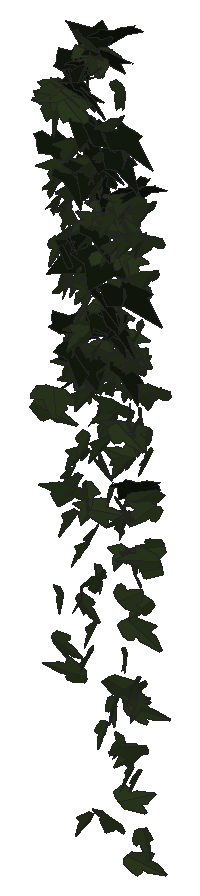
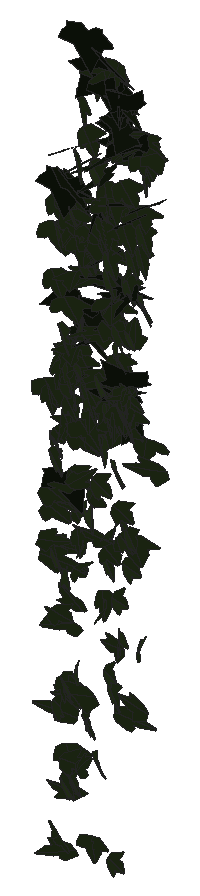
# SketchUp Ruby script. Lengths in millimetres.
U = 1.mm
M = Sketchup.active_model
def pt(a) = Geom::Point3d.new(a.map { |v| v * U })
def face(e, loops, mat)
  f = e.add_face(loops[0].map { |a| pt(a) })
  loops[1..].each { |l| e.add_face(l.map { |a| pt(a) }).erase! }
  f.material = f.back_material = mat if mat
  f
end
# faces: each face lists its corners as indices into pts; further lists are holes
def faces(e, pts, list, mat = nil) = list.each { |f| face(e, (f[0].is_a?(Array) ? f : [f]).map { |l| l.map { |i| pts[i] } }, mat) }
# xy, xz, yz: faces in a plane at the given z, y or x. An outline is a flat list of corners, or four numbers for a rectangle; further outlines are holes
def ring(l) = l.size == 4 ? [[l[0], l[1]], [l[2], l[1]], [l[2], l[3]], [l[0], l[3]]] : l.each_slice(2).to_a
def flat(e, list, mat, &to3) = list.each { |f| face(e, (f[0].is_a?(Array) ? f : [f]).map { |l| ring(l).map { |u, v| to3.(u, v) } }, mat) }
def xy(e, z, list, mat = nil) = flat(e, list, mat) { |x, y| [x, y, z] }
def xz(e, y, list, mat = nil) = flat(e, list, mat) { |x, z| [x, y, z] }
def yz(e, x, list, mat = nil) = flat(e, list, mat) { |y, z| [x, y, z] }
def lines(e, pts, list) = list.each { |a, b| e.add_line(pt(pts[a]), pt(pts[b])) }
# prism: a flat outline (further loops are holes) pulled along v
def prism(e, loops, v, mat = nil)
  f = face(e, loops, mat); d = Geom::Vector3d.new(v.map { |x| x * U })
  f.pushpull(f.normal.samedirection?(d) ? d.length : -d.length)
end
def box(e, o, s, mat = nil) = prism(e, [[o, [o[0] + s[0], o[1], o[2]], [o[0] + s[0], o[1] + s[1], o[2]], [o[0], o[1] + s[1], o[2]]]], [0, 0, s[2]], mat)
def at(x, y, z, deg = 0) = Geom::Transformation.translation(pt([x, y, z])) * Geom::Transformation.rotation(ORIGIN, Z_AXIS, deg.degrees)
def axes(o, x, y, z) = Geom::Transformation.new([*x, 0, *y, 0, *z, 0, *pt(o).to_a, 1])
def part(name) = M.definitions.add(name)
# library, detail: a bought-in or finely detailed component or shape, given as its bounding box
def library(name, o, s) = part(name).tap { |d| box(d.entities, o, s) }
def detail(e, o, s) = box(e.add_group.entities, o, s)
def put(e, d, t, mat = nil) = e.add_instance(d, t).tap { |i| i.material = mat if mat }
def group(e, t, mat = nil) = e.add_group.tap { |g| g.transformation = t; g.material = mat if mat }.entities
root = M.entities
M.materials.add("efeu1").color = [18, 25, 13]
M.materials.add("efeu2").color = [43, 57, 29]
c1 = part("ivyleaf_10")
p = [[0,12.8,-0.8],[-1.5,51.3,-10.9],[-4.9,51,-11.6],[-13.6,26.5,-7.3],[-13.2,15.9,-4.6],[-21.1,19.3,-7.2],
  [-29.5,16.3,-8.3],[-29.2,8.3,-6.2],[-19.7,-9.8,0.5],[-7.6,-13,4],[1,-12.2,5.8],[-0.4,51.1,-11.1],
  [-1.5,51.1,-10.9],[1,-12.4,5.9],[16.9,-12.4,3.5],[35.1,9.1,-5.1],[35,12.9,-6.1],[20.5,16.4,-4.9],
  [15.8,15,-3.8],[15.3,27.6,-7.1],[12.8,31.3,-7.8]]
faces(c1.entities,p,[[0,1,2,3,4,5,6,7,8,9,10],[11,12,0,13,14,15,16,17,18,19,20]],"efeu2")
c2 = part("ivyleaf_9")
p = [[39.1,54.8,31.7],[34.5,51.8,30.2],[-5.3,25.2,17.3],[-17.9,28.3,20.9],[-21.6,21.7,17],[-20.2,4.3,5.3],
  [-22.9,-0.3,2.5],[-17.1,-4,-0.6],[-2,-2.1,-1.2],[-0.7,-15.4,-10.1],[16.6,-22.3,-16.7],[21.1,-15.1,-12.5],
  [32.7,-10.7,-11],[46.1,-1.8,-6.6],[30.8,11.2,3.8]]
faces(c2.entities,p,[[0,1,2,3,4,5,6,7,8,9,10,11,12,13,14]],"efeu1")
put(root,c1,axes([1236.6,996.8,859],[-0.48434,-0.01854,-0.67596],[1.27265,-0.11431,-0.24861],[-0.1914,-0.71317,0.05742]))
put(root,c1,axes([1267.7,996.5,1433.3],[-0.73071,-0.64843,0.24389],[-0.04626,-0.26606,-0.74563],[1.31768,-0.36892,0.10907]))
put(root,c1,axes([1262.1,1002.8,1162.8],[0.77658,-0.63464,0.15423],[0.15396,-0.13134,-0.75449],[1.23344,0.41597,-0.00293]))
put(root,c2,axes([1251,1002.6,1352.9],[0.2551,-0.72169,-0.24865],[0.08886,0.25974,-0.72869],[1.45004,0.11105,0.0884]))
put(root,c1,axes([1269.6,998,1254.6],[0.07758,-0.76332,-0.07843],[0.03185,0.0794,-0.76412],[1.46005,0.03882,0.02083]))
put(root,c1,axes([1278.6,1010,717.3],[-1.12301,-0.45413,0.18457],[-0.24328,-0.1363,-0.74402],[0.90069,-0.60305,0.02917]))
put(root,c1,axes([1272.7,990.3,1291.2],[-0.0053,-0.76905,0.00236],[-0.00122,-0.00236,-0.76906],[1.46367,-0.00279,-0.00063]))
put(root,c1,axes([1247.8,1026.8,420],[-0.05358,0.0607,-0.71661],[0.97993,-0.499,-0.06249],[-0.95561,-0.5151,-0.0239]))
put(root,c1,axes([1270.7,1026.9,740.1],[0.12388,-0.62126,0.15416],[0.10876,-0.1487,-0.62337],[1.21338,0.07676,0.04014]))
put(root,c1,axes([1270.5,987.4,1404.9],[0.66757,-0.69995,-0.15253],[0.11635,0.19846,-0.77014],[1.35844,0.32697,0.14092]))
put(root,c1,axes([1285.4,992.2,1461.8],[1.00596,0.26839,-0.54166],[-0.95,-0.21209,-0.59217],[-0.64897,0.7265,0.02723]))
put(root,c1,axes([1297.6,1010.7,384.3],[-0.04672,-0.00322,0.68376],[-1.24545,-0.19826,-0.02443],[0.3773,-0.65485,0.00403]))
put(root,c1,axes([1255.8,994,1442.4],[-0.97704,-0.15716,-0.58973],[1.10384,0.11426,-0.53534],[0.36159,-0.77348,0.04075]))
put(root,c1,axes([1265.2,986.9,897.9],[1.3992,0.19283,0.10718],[0.18718,0.04733,-0.75977],[-0.37585,0.74144,0.02063]))
put(root,c1,axes([1264.9,1007.9,514.3],[-0.18596,-0.0466,0.72839],[0.74159,-0.62473,0.0123],[1.17458,0.38705,0.10756]))
put(root,c1,axes([1277,1007.8,1090.6],[-0.35052,-0.6667,-0.28883],[-0.17614,-0.27401,0.69151],[-1.37156,0.20558,-0.01499]))
put(root,c1,axes([1282.5,1020.9,948.5],[0.50606,-0.62103,-0.12277],[-0.07777,0.11604,-0.67551],[1.20231,0.2689,0.00798]))
put(root,c1,axes([1285.2,988.6,1322.2],[-0.86934,-0.61046,0.15935],[-0.01235,-0.19217,-0.75481],[1.2007,-0.44397,0.10761]))
put(root,c1,axes([1282.6,1027.7,729],[0.00113,-0.57979,0.27924],[0.05888,-0.27889,-0.57913],[1.22335,0.01396,0.02762]))
put(root,c1,axes([1281.4,1000.5,949.3],[0.20567,-0.46714,-0.52578],[0.14616,0.53661,-0.46098],[1.33057,0.01326,0.13191]))
put(root,c1,axes([1285.9,1001.7,1249.9],[-0.02219,-0.75998,-0.05861],[0.01802,0.05847,-0.76002],[1.45058,-0.01235,0.00854]))
put(root,c1,axes([1285.1,992.2,1459.4],[1.24855,0.43136,-0.17251],[-0.39567,0.00564,-0.7765],[-0.79071,0.67831,0.11616]))
put(root,c1,axes([1288.1,1008.4,1199.9],[-0.03972,-0.74212,-0.0126],[-0.00115,0.01262,-0.74241],[1.41261,-0.02086,-0.00096]))
put(root,c1,axes([1285.7,1012.2,668.7],[0.12431,-0.5106,0.52642],[0.19752,-0.51675,-0.5141],[1.3817,0.11981,0.02613]))
put(root,c1,axes([1291.2,1029.3,781.1],[-0.17924,-0.53573,0.39099],[-0.05732,-0.39105,-0.54307],[1.26097,-0.09393,0.03089]))
put(root,c1,axes([1280.5,1014.4,1107.4],[0.30435,-0.46144,0.60436],[0.46387,-0.55388,-0.4874],[1.37079,0.28989,0.03075]))
put(root,c1,axes([1291.8,1013.3,955.6],[-1.04393,-0.48159,-0.06748],[0.10188,0.04131,-0.72992],[0.9199,-0.5511,0.00426]))
put(root,c1,axes([1291.3,1005.5,975.5],[0.34361,-0.4942,-0.48629],[-0.00492,0.50203,-0.51115],[1.31955,0.13056,0.12472]))
put(root,c1,axes([1289.1,994.5,1234.4],[0.18803,-0.5842,-0.47304],[0.28392,0.48285,-0.56517],[1.40218,-0.01943,0.17787]))
put(root,c1,axes([1315,1007.3,986.2],[-0.75242,-0.02108,0.59441],[-1.09376,-0.1704,-0.38827],[0.29172,-0.69324,0.07736]))
put(root,c2,axes([1289.2,998.2,1185.1],[1.01041,-0.23892,-0.52743],[-0.86423,0.27219,-0.58038],[0.68375,0.69711,0.04585]))
put(root,c1,axes([1287.1,1007.1,992.1],[0.15937,-0.06374,0.73173],[0.0287,0.73646,0.06242],[-1.3976,0.00786,0.08472]))
put(root,c2,axes([1298,983.1,925.4],[0.26957,0.57002,0.50842],[0.24425,0.49198,-0.58734],[-1.43303,0.19108,-0.00447]))
put(root,c1,axes([1297.4,1009.4,737.9],[0.35226,-0.59652,-0.18005],[-0.02889,0.18345,-0.6234],[1.18554,0.18172,0.03831]))
put(root,c1,axes([1296.6,1019.9,965.4],[0.406,-0.6716,0.06352],[0.02866,-0.06187,-0.70465],[1.28357,0.21381,-0.00436]))
put(root,c1,axes([1300.5,999,1285.3],[-0.2733,-0.7494,0.01594],[-0.01021,-0.0152,-0.76303],[1.42655,-0.14368,-0.00241]))
put(root,c1,axes([1300,1019.5,1109.2],[0.02503,-0.67465,0.2926],[0.03464,-0.29226,-0.67469],[1.39914,0.01931,0.01147]))
put(root,c1,axes([1308.9,1011.7,980.1],[-0.46867,0.52454,-0.45681],[-0.36459,0.4147,0.57947],[1.27261,0.31198,-0.00222]))
put(root,c2,axes([1287.3,1009.8,1009.3],[-0.69557,-0.07879,0.68714],[1.27312,0.15724,0.37382],[-0.33453,0.76224,-0.00609]))
put(root,c2,axes([1301.2,990.1,1476.8],[0.62333,0.64045,0.36642],[0.0415,0.39232,-0.70521],[-1.40368,0.296,0.14186]))
put(root,c1,axes([1305.4,997.2,1365.4],[-0.52946,-0.69054,0.23758],[-0.07237,-0.24019,-0.74266],[1.38796,-0.27594,0.0519]))
put(root,c1,axes([1298.2,1026.1,608.2],[0.13264,-0.43926,0.49745],[0.19787,-0.48679,-0.44441],[1.24744,0.12392,0.0176]))
put(root,c1,axes([1300.2,1006.7,989.5],[0.0641,-0.16022,0.69276],[-0.27177,0.67788,0.16372],[-1.3257,-0.14672,-0.00007]))
put(root,c2,axes([1321,997.8,1195.3],[-0.81049,0.61854,0.11361],[-0.09102,0.10495,-0.7507],[-1.19344,-0.42807,-0.0199]))
put(root,c1,axes([1301.8,1016,928],[-1.11684,-0.40969,-0.16454],[0.27417,0.08102,-0.71552],[0.79426,-0.60405,0.01563]))
put(root,c1,axes([1306.2,1005.1,528.2],[0.0608,-0.47522,-0.52635],[-0.0232,0.52644,-0.47603],[1.34943,0.03046,0.01553]))
put(root,c2,axes([1292.6,1002.4,1307.7],[-0.06609,-0.77013,0.0127],[-0.0186,-0.01227,-0.77086],[1.4658,-0.03488,-0.00921]))
put(root,c1,axes([1307.3,1016,940.5],[-0.04105,-0.61766,-0.40572],[0.05295,0.40493,-0.61793],[1.40547,-0.03329,0.01143]))
put(root,c1,axes([1305.6,1027.5,116.3],[0.02412,-0.5141,0.4136],[0.1196,-0.41086,-0.51261],[1.25006,0.04923,0.04106]))
put(root,c2,axes([1295.7,989.2,1471],[1.47071,0.15477,-0.17109],[-0.32731,-0.01221,-0.78782],[-0.29267,0.79138,0.02131]))
put(root,c2,axes([1282.1,993,1451.1],[1.02002,-0.52969,0.2753],[0.43293,-0.16085,-0.75232],[1.05041,0.58066,0.04274]))
put(root,c2,axes([1296.9,996.5,1168.3],[0.55199,-0.61027,-0.36689],[-0.19549,0.35616,-0.67361],[1.34103,0.30312,0.05282]))
put(root,c2,axes([1303.6,987.9,1510.1],[-0.44831,-0.17537,0.75681],[1.161,0.44791,0.29366],[-0.91546,0.65392,0.00181]))
put(root,c2,axes([1307.4,1008.5,980.3],[-0.46016,-0.73558,0.02858],[-0.01743,-0.02707,-0.7743],[1.4009,-0.24196,-0.00025]))
put(root,c1,axes([1316.2,1025.1,692.7],[-0.46916,-0.50319,0.3595],[0.05123,-0.39538,-0.53494],[1.17586,-0.18355,0.16675]))
put(root,c2,axes([1326.4,998.3,1163.9],[-1.02599,-0.43006,0.3961],[-0.5662,-0.26206,-0.68941],[0.95795,-0.6155,0.01676]))
put(root,c1,axes([1316.3,1017.5,1152.3],[-1.0997,-0.47349,0.0296],[0.17302,-0.15629,-0.72543],[0.88618,-0.55707,0.17837]))
put(root,c1,axes([1303.7,982.4,1439.8],[0.48291,0.68445,0.326],[0.26394,0.29607,-0.72955],[-1.41851,0.2881,-0.02476]))
put(root,c1,axes([1320.2,998.4,1036.4],[-0.44478,-0.68713,0.08115],[-0.0293,-0.08047,-0.72569],[1.3165,-0.23394,0.01127]))
put(root,c1,axes([1319.1,1012.4,427.6],[0.25523,-0.72065,0.02541],[0.0055,-0.02531,-0.73302],[1.37239,0.13412,-0.00179]))
put(root,c1,axes([1300.8,1019.3,514.9],[-0.42315,0.17606,-0.62368],[0.74416,-0.48939,-0.27754],[-0.9836,-0.446,0.05834]))
put(root,c2,axes([1338.2,975,1513.4],[-0.2612,0.71433,0.35682],[-0.47322,0.30582,-0.70786],[-1.44412,-0.22941,0.16742]))
put(root,c1,axes([1314.8,1028.5,467],[0.19969,-0.48968,0.41911],[0.27712,-0.39564,-0.49871],[1.19498,0.17358,0.04562]))
put(root,c1,axes([1300.5,1017.2,925.4],[0.66729,-0.25449,0.59573],[0.92461,-0.34481,-0.43323],[0.81559,0.59911,0.00372]))
put(root,c1,axes([1322.6,1015,1234.7],[0.02751,-0.74954,0.00252],[0.00026,-0.00251,-0.74968],[1.42654,0.01445,0.00009]))
put(root,c1,axes([1314.8,1014.9,730],[0.03351,0.63966,-0.25407],[-0.00429,-0.2541,-0.63989],[-1.30992,0.0172,-0.0044]))
put(root,c2,axes([1333.8,985.6,1529.5],[0.20841,0.02188,-0.80908],[-1.38345,0.36171,-0.0886],[0.67742,0.73196,0.06797]))
put(root,c1,axes([1312.2,1006.4,1050.5],[0.72044,-0.52663,0.45237],[0.47326,-0.37821,-0.64838],[1.23364,0.45265,-0.01545]))
put(root,c1,axes([1327.9,1011.2,1104.2],[-0.3751,-0.57925,0.37893],[-0.1767,-0.36831,-0.6113],[1.30546,-0.21629,0.02614]))
put(root,c1,axes([1323.5,998.7,1026.2],[-0.16443,-0.47363,0.62044],[0.07269,-0.62605,-0.47259],[1.48378,-0.02182,0.09191]))
put(root,c1,axes([1326.8,1012.3,946.8],[0.03882,-0.7307,-0.24751],[-0.0407,0.24696,-0.73085],[1.46771,0.02617,-0.01372]))
put(root,c1,axes([1329.7,1007.8,1331.1],[-1.09721,-0.47267,0.17984],[-0.05766,-0.23995,-0.72775],[0.96077,-0.55419,0.16171]))
put(root,c1,axes([1322.4,998.5,830.8],[0.7332,-0.56711,0.15923],[0.14428,-0.14094,-0.6854],[1.11174,0.3923,-0.01606]))
put(root,c2,axes([1318.1,998.9,1417.5],[-0.37113,-0.71034,0.27755],[-0.01133,-0.28505,-0.73372],[1.4514,-0.18386,0.06524]))
put(root,c1,axes([1328.7,1008.4,1198.1],[0.04597,-0.75249,-0.05337],[0.00466,0.05347,-0.75287],[1.43573,0.02392,0.00415]))
put(root,c1,axes([1334.6,1002.8,946.2],[0.89717,-0.25713,-0.48283],[-0.39415,0.50605,-0.47168],[0.96361,0.44639,0.25661]))
put(root,c1,axes([1310.2,1004.8,1137.7],[0.64613,-0.32668,0.58534],[0.92177,-0.33408,-0.46736],[0.88201,0.58845,0.05962]))
put(root,c2,axes([1319.1,1006.8,982],[-0.65523,-0.58416,-0.37826],[0.39536,0.31651,-0.67788],[1.26412,-0.40178,0.01595]))
put(root,c1,axes([1334.1,995,920.5],[-0.21296,-0.7104,0.25282],[-0.08054,-0.24927,-0.71915],[1.43284,-0.1196,-0.00285]))
put(root,c1,axes([1328,1006.6,1129.4],[-0.13197,0.45006,0.60166],[0.2609,-0.5865,0.45451],[1.40599,0.15107,-0.02787]))
put(root,c1,axes([1331.7,985.7,1523.5],[0.39125,-0.71692,-0.33425],[0.00518,0.34599,-0.74043],[1.50544,0.18513,0.08941]))
put(root,c2,axes([1309.2,990.4,1489.5],[0.7734,-0.68843,0.09577],[0.06844,-0.08997,-0.79928],[1.32106,0.40769,-0.01466]))
put(root,c1,axes([1333.3,1007,659.4],[0.14814,-0.63698,0.05729],[0.02649,-0.05602,-0.64168],[1.2169,0.07876,0.00699]))
put(root,c1,axes([1333,989.6,1088.2],[0.53261,-0.70127,0.0322],[0.01506,-0.03151,-0.75503],[1.33598,0.27993,-0.00432]))
put(root,c1,axes([1331,1005.2,949.5],[-0.45935,-0.64895,-0.38243],[0.35652,0.33725,-0.69051],[1.38854,-0.30128,0.05078]))
put(root,c1,axes([1327.7,1024.3,579],[-0.12561,0.58529,-0.36019],[0.07722,-0.3579,-0.589],[-1.30568,-0.07747,-0.00018]))
put(root,c2,axes([1341,983.9,1541.1],[0.31889,0.79739,-0.08508],[-0.03436,-0.08314,-0.8148],[-1.52581,0.16852,0.00057]))
put(root,c1,axes([1337.8,980.2,1570.8],[-1.26706,0.4666,0.12122],[-0.19505,0.06497,-0.81297],[-0.89655,-0.67357,0.00555]))
put(root,c1,axes([1337.4,1027.4,813.9],[0.01221,-0.60134,0.43483],[0.06009,-0.43423,-0.60098],[1.41105,0.02369,0.02183]))
put(root,c1,axes([1335.9,1011.5,1289.6],[1.09486,-0.43649,-0.23143],[-0.08284,0.30907,-0.69109],[0.93661,0.53757,0.20941]))
put(root,c1,axes([1335.7,1003.3,1329.3],[0.47299,-0.70335,-0.22325],[0.10687,0.25291,-0.73429],[1.40035,0.21826,0.13144]))
put(root,c1,axes([1339,1017.8,998.8],[0.22659,-0.72023,0.14581],[0.00543,-0.14726,-0.72971],[1.39855,0.11726,-0.02079]))
put(root,c2,axes([1336.7,1007.9,1324.7],[-0.8685,-0.62023,0.03577],[0.04951,-0.06342,-0.76779],[1.18135,-0.45332,0.05848]))
put(root,c1,axes([1341.9,1009.7,883.2],[0.18117,-0.68907,-0.31051],[-0.06661,0.3086,-0.69558],[1.43689,0.10118,0.00691]))
put(root,c2,axes([1363,979.6,1573.9],[-0.44183,0.48026,0.63359],[-0.59948,0.55048,-0.53267],[-1.38929,-0.39026,0.02835]))
put(root,c1,axes([1355.3,997.5,1240.2],[-0.56364,-0.45272,0.59647],[-0.59231,-0.50899,-0.54084],[1.29624,-0.42943,0.01222]))
put(root,c1,axes([1336.3,1028.9,292.6],[0.65999,-0.51478,0.30275],[0.30412,-0.25734,-0.62061],[1.09516,0.38169,-0.01011]))
put(root,c1,axes([1346.9,992.8,1347],[-0.30835,-0.75138,-0.14465],[0.03071,0.14447,-0.76851],[1.45595,-0.16218,-0.01443]))
put(root,c1,axes([1350.7,997.3,1251.6],[0.63491,-0.50102,-0.47557],[-0.24126,0.47475,-0.58908],[1.29237,0.33477,0.12367]))
put(root,c1,axes([1347.4,998.2,584.1],[-0.23384,-0.7097,-0.14698],[0.07533,0.14228,-0.72011],[1.3773,-0.12828,0.01443]))
put(root,c2,axes([1353.9,985.6,1303.7],[0.59075,-0.10777,-0.72803],[-1.26929,0.29293,-0.32771],[0.5923,0.73523,0.02385]))
put(root,c1,axes([1355.8,1019.7,133.5],[-1.11755,0.14148,0.21251],[-0.40192,0.03031,-0.6037],[-0.27302,-0.62373,0.01887]))
put(root,c1,axes([1352.9,992.9,1308.6],[0.38599,-0.74123,0.10891],[0.04804,-0.106,-0.76847],[1.42505,0.20435,-0.00359]))
put(root,c2,axes([1339.8,1005.2,1224.5],[0.08373,-0.75772,-0.04526],[-0.01507,0.04488,-0.75897],[1.44458,0.04439,-0.00529]))
put(root,c1,axes([1357,1023.5,964.7],[-0.10265,-0.6894,0.01608],[-0.00424,-0.01596,-0.6915],[1.31241,-0.05397,-0.00098]))
put(root,c1,axes([1360.5,1009.9,771.5],[-0.97111,0.54537,-0.05767],[-0.07594,0.04165,0.74685],[1.04096,0.51181,0.00068]))
put(root,c1,axes([1339.3,1006,1001],[-0.6967,-0.22679,-0.57957],[0.95417,0.29093,-0.43051],[0.70181,-0.62069,0.00997]))
put(root,c1,axes([1346.9,983.8,1556.1],[1.15875,0.5261,0.15581],[0.17913,0.12915,-0.80387],[-1.02878,0.61505,0.03552]))
put(root,c1,axes([1355.8,983.1,1549.1],[0.09512,0.77008,0.28288],[-0.21089,0.28714,-0.76212],[-1.54707,0.00821,0.12128]))
put(root,c1,axes([1360.3,1017.7,937],[-0.19961,-0.6501,-0.24321],[0.10356,0.23752,-0.65834],[1.31696,-0.11721,0.0149]))
put(root,c1,axes([1376.1,1014.6,900.3],[-1.11307,-0.21196,0.36112],[-0.64939,-0.11833,-0.62205],[0.46193,-0.67709,-0.00433]))
put(root,c1,axes([1352.9,1025.8,729.7],[-0.11519,-0.22027,-0.66498],[0.18138,-0.66384,0.21122],[-1.32082,-0.07195,0.087]))
put(root,c1,axes([1335.4,1009.5,698.8],[0.28326,-0.18809,-0.62528],[1.21612,-0.08999,0.17916],[-0.25567,-0.63642,0.15947]))
put(root,c2,axes([1347,984.7,1371],[0.94144,-0.49057,-0.37121],[-0.33622,0.34299,-0.68869],[1.12151,0.51463,0.10514]))
put(root,c1,axes([1371.6,1005.2,1265.4],[-0.90169,-0.43475,0.39921],[-0.26022,-0.41715,-0.61655],[1.09278,-0.45806,0.18259]))
put(root,c2,axes([1344.6,1003,1403.3],[0.59673,-0.67539,-0.23782],[0.0089,0.26155,-0.7366],[1.36273,0.29404,0.10895]))
put(root,c2,axes([1366.6,995.5,1175],[-0.96627,-0.58128,0.01043],[-0.01891,-0.00518,-0.77177],[1.1063,-0.50779,-0.00408]))
put(root,c1,axes([1370.4,1018.5,965],[0.84304,-0.54735,-0.35738],[-0.31096,0.3253,-0.70073],[1.20463,0.46703,0.06922]))
put(root,c1,axes([1366.9,1005.6,881],[-0.21509,-0.63831,0.27205],[0.06876,-0.28067,-0.64353],[1.31877,-0.08947,0.07793]))
put(root,c2,axes([1370.9,984.6,1305.8],[0.30168,-0.09878,-0.78481],[-1.09877,0.5327,-0.18365],[1.02908,0.59773,0.03398]))
put(root,c1,axes([1369.1,992.9,1377.1],[0.16313,-0.76934,0.19742],[0.03664,-0.19649,-0.77409],[1.5112,0.08781,-0.00254]))
put(root,c1,axes([1366.5,1020.4,987.1],[0.05054,-0.66266,0.30431],[0.19186,-0.29825,-0.65827],[1.37448,0.066,0.0807]))
put(root,c2,axes([1356,981.1,1559.3],[1.46253,0.28256,-0.05523],[-0.1289,0.02441,-0.81746],[-0.53257,0.77005,0.04618]))
put(root,c1,axes([1347.9,1004.4,1079.7],[-0.42066,-0.26492,-0.64104],[1.16582,0.24108,-0.31084],[0.6193,-0.63377,0.14972]))
put(root,c2,axes([1351.4,1002,1100.7],[0.32585,-0.66389,0.41643],[0.27209,-0.39264,-0.68474],[1.46648,0.22037,0.03452]))
put(root,c1,axes([1377.9,1004.1,1250.9],[-0.45654,-0.65077,0.29698],[-0.10859,-0.29483,-0.69214],[1.35709,-0.24252,0.04452]))
put(root,c1,axes([1374.4,1006.3,1228.8],[0.55793,-0.70256,0.01967],[0.01201,-0.01868,-0.76127],[1.33758,0.29322,-0.00137]))
put(root,c1,axes([1368.8,1017.7,354.9],[0.48048,-0.61681,0.30711],[0.31169,-0.26399,-0.66483],[1.27379,0.29726,0.04683]))
put(root,c1,axes([1368.5,1030.4,270],[-0.03496,0.05324,0.71324],[0.45298,-0.67236,0.05632],[1.28363,0.23872,-0.00045]))
put(root,c2,axes([1394.1,991,1063.7],[-0.81984,0.62259,0.10496],[-0.13601,0.07817,-0.75695],[-1.19391,-0.43643,0.01415]))
put(root,c1,axes([1362.4,1019.4,351.3],[0.62915,-0.40707,0.46381],[0.64813,-0.31845,-0.52222],[0.97945,0.47221,0.04764]))
put(root,c1,axes([1378.9,1008,1239.4],[-1.00105,-0.52412,-0.07313],[0.13774,0.03089,-0.74197],[0.9977,-0.53014,0.02906]))
put(root,c1,axes([1382.3,1030.2,800.8],[0.15455,0.42894,0.55127],[-0.15849,-0.54508,0.43639],[1.31989,-0.11568,-0.01215]))
put(root,c1,axes([1381.1,1003.3,1203.1],[0.00519,-0.64219,0.39214],[0.04466,-0.39188,-0.64193],[1.43137,0.01456,0.0186]))
put(root,c2,axes([1367.4,990.1,1068.3],[0.21549,-0.65761,-0.38062],[-0.15508,0.3721,-0.66712],[1.43775,0.1387,-0.01491]))
put(root,c1,axes([1371.9,1025.8,687.9],[-0.12862,0.31516,-0.62508],[0.18984,-0.61725,-0.32199],[-1.31872,-0.11959,0.01461]))
put(root,c1,axes([1382.7,1018.6,696.9],[-0.23233,-0.67095,-0.14265],[0.06358,0.1389,-0.68192],[1.30394,-0.12632,0.00783]))
put(root,c1,axes([1393.8,1005.7,871.9],[-0.5821,-0.44508,0.40869],[-0.46451,-0.32803,-0.5399],[1.05202,-0.39111,-0.01226]))
put(root,c2,axes([1369.6,999.8,1062.9],[0.18171,-0.75103,-0.16729],[-0.05666,0.16484,-0.75703],[1.4633,0.09965,-0.00854]))
put(root,c1,axes([1387.7,992.3,1436.3],[-0.22092,-0.78207,0.08337],[-0.03162,-0.08182,-0.79062],[1.49653,-0.11718,-0.0044]))
put(root,c1,axes([1366.1,993.4,1179.3],[0.82035,0.49262,0.46939],[0.58797,0.35339,-0.65457],[-1.15384,0.53032,0.00017]))
put(root,c1,axes([1382.2,1022,632.8],[-0.3295,-0.38144,0.48849],[0.27582,-0.51805,-0.35316],[1.14685,0.015,0.22528]))
put(root,c1,axes([1386,1016.1,997],[0.60689,-0.67068,0.08663],[0.05901,-0.08118,-0.74259],[1.28568,0.32031,-0.00681]))
put(root,c1,axes([1404.5,1007.8,945.4],[0.06772,-0.05301,0.75932],[-0.93491,0.57906,0.06344],[-1.10659,-0.49247,-0.00713]))
put(root,c1,axes([1395.1,1014.5,806.5],[-0.15075,-0.57044,0.38723],[-0.03947,-0.38763,-0.57527],[1.31157,-0.07723,0.0272]))
put(root,c2,axes([1398.4,976,1614],[0.51204,0.77907,-0.13785],[-0.08069,-0.1312,-0.82421],[-1.50359,0.27235,-0.00271]))
put(root,c1,axes([1381.8,1026.4,437.8],[0.01596,-0.05996,0.64957],[0.70857,-0.53299,-0.05401],[1.01947,0.37139,0.02737]))
put(root,c1,axes([1395.3,999.2,1073.8],[0.32039,-0.33193,-0.63703],[0.09444,0.6581,-0.32979],[1.36384,0.0324,0.17249]))
put(root,c1,axes([1398.6,1024.7,945.2],[-0.16642,-0.66797,0.14057],[0.03158,-0.14375,-0.6728],[1.29875,-0.0821,0.03437]))
put(root,c1,axes([1404.5,1023.7,1126.9],[-1.06979,-0.38238,0.26694],[-0.15395,-0.33178,-0.6456],[0.87407,-0.52643,0.213]))
put(root,c1,axes([1401.8,1025.7,270.3],[-0.15574,-0.34307,0.6304],[-0.02048,-0.63382,-0.34633],[1.36578,-0.04862,0.06669]))
put(root,c1,axes([1398.5,1018,237.3],[0.41345,-0.6449,0.15211],[0.08451,-0.14555,-0.68049],[1.25822,0.22169,-0.00428]))
put(root,c1,axes([1375.3,1010.5,394.4],[-0.63433,0.06564,-0.65922],[1.24484,-0.08457,-0.33911],[-0.2002,-0.73383,-0.01989]))
put(root,c1,axes([1399.2,992.2,1496.4],[0.88416,-0.6346,-0.16218],[0.04433,0.21472,-0.77343],[1.24581,0.44274,0.14262]))
put(root,c1,axes([1428.1,994.6,1240.6],[-0.43475,0.05655,0.74398],[-1.40849,-0.11613,-0.2184],[0.18061,-0.76954,0.08763]))
put(root,c1,axes([1405.4,990.9,1120.3],[0.37124,-0.62436,-0.44065],[-0.13018,0.43869,-0.65186],[1.44859,0.19943,0.05435]))
put(root,c1,axes([1403.5,1019.6,1000],[-0.03397,-0.71046,-0.12065],[0.02157,0.1204,-0.71063],[1.37133,-0.01949,0.00819]))
put(root,c1,axes([1406.6,1008.6,1281.2],[-0.56548,-0.70174,0.08196],[-0.04772,-0.07839,-0.76201],[1.34378,-0.29808,0.00743]))
put(root,c1,axes([1395.4,1013.6,1178.9],[0.57522,0.67377,0.01159],[0.00207,0.01222,-0.73844],[-1.2825,0.30222,0.00401]))
put(root,c1,axes([1395.2,1010.7,1038.5],[0.83995,0.54897,0.06696],[0.0067,0.08287,-0.70267],[-1.05253,0.43862,0.04896]))
put(root,c1,axes([1400,1032.9,979.3],[0.06702,-0.27822,0.64107],[0.22614,-0.63015,-0.28001],[1.31066,0.12295,0.01553]))
put(root,c1,axes([1407.7,998.9,1011],[-0.8467,-0.62171,0.01663],[-0.01521,-0.01472,-0.76448],[1.18356,-0.44495,0.00207]))
put(root,c2,axes([1384.2,993.4,1070.2],[0.51049,-0.71704,0.18582],[0.07826,-0.18291,-0.76517],[1.40758,0.27022,-0.02485]))
put(root,c1,axes([1408.6,1013.8,282.7],[-0.75027,-0.632,0.01407],[-0.00852,-0.0138,-0.74486],[1.20309,-0.39423,0.0035]))
put(root,c1,axes([1401.1,1002.8,1263.2],[0.32699,0.63478,0.40598],[-0.07788,0.42365,-0.64508],[-1.43195,0.12191,0.12779]))
put(root,c1,axes([1407.1,1002.5,1237.1],[-0.84309,0.6305,0.26282],[0.22027,-0.23944,0.76949],[1.28125,0.45604,0.04065]))
put(root,c1,axes([1405.5,1027.2,228.6],[0.41461,-0.64846,0.29497],[0.17401,-0.28045,-0.68407],[1.34462,0.23625,-0.00243]))
put(root,c1,axes([1422.4,1006.1,610.3],[-0.18447,0.07568,0.7615],[-0.97228,0.5651,-0.12118],[-1.08436,-0.51956,-0.02089]))
put(root,c1,axes([1410.4,988.6,1382.9],[0.54326,-0.66525,-0.30561],[-0.08094,0.3124,-0.71975],[1.39097,0.278,0.07748]))
put(root,c1,axes([1410.8,997.4,1285.1],[0.27723,-0.76213,-0.00746],[-0.00467,0.00712,-0.77593],[1.45056,0.14568,-0.00107]))
put(root,c2,axes([1394.2,989.6,1377.9],[0.36285,-0.74802,-0.1562],[-0.01027,0.15966,-0.77121],[1.45431,0.18776,0.03352]))
put(root,c2,axes([1395.6,1008.9,980],[0.13381,-0.75365,0.20487],[0.07698,-0.20191,-0.75663],[1.4844,0.07841,0.02077]))
put(root,c2,axes([1392.1,997.5,1415.9],[0.44839,-0.67759,-0.31851],[0.15769,0.35545,-0.69489],[1.41621,0.17495,0.17822]))
put(root,c1,axes([1424.2,984.6,900.7],[-0.27364,0.1965,0.73988],[-0.79073,0.61227,-0.24335],[-1.22371,-0.43957,-0.0082]))
put(root,c1,axes([1421.2,992.1,1305],[-0.99368,-0.50137,0.25286],[-0.17535,-0.2641,-0.71391],[1.05421,-0.51651,0.11959]))
put(root,c1,axes([1395.1,1008.1,555.6],[0.96527,-0.21012,-0.38853],[0.67555,-0.15822,0.54892],[-0.50034,-0.619,-0.00842]))
put(root,c1,axes([1396.3,1001.6,723.2],[-0.45786,-0.00862,0.63768],[1.01155,-0.37936,0.19539],[0.67076,0.56621,0.14061]))
put(root,c1,axes([1419.6,1000.3,1230.6],[-0.22463,-0.65996,0.36858],[-0.0548,-0.36885,-0.66966],[1.4376,-0.11718,0.03207]))
put(root,c1,axes([1419.7,1032.4,545.8],[-0.32462,-0.41151,0.50788],[-0.0371,-0.52144,-0.42905],[1.2435,-0.12298,0.11978]))
put(root,c1,axes([1414.9,1013,407.7],[0.39132,-0.66087,0.29802],[0.19706,-0.27983,-0.69196],[1.36559,0.22975,0.01445]))
put(root,c1,axes([1445.4,1015.3,634.4],[0.17432,0.0185,-0.7632],[-1.42839,0.14293,-0.0866],[0.26604,0.75527,0.03508]))
put(root,c2,axes([1428.7,998,784.2],[0.30423,0.64181,-0.39188],[-0.23283,-0.3731,-0.66096],[-1.41213,0.19979,0.02455]))
put(root,c1,axes([1420.9,1007.2,404.6],[-0.3624,-0.63364,-0.10714],[0.08569,0.09831,-0.66148],[1.22006,-0.19512,0.01463]))
put(root,c1,axes([1419.2,1015.6,998.4],[-0.41383,-0.6239,-0.26462],[0.23828,0.23614,-0.65963],[1.26759,-0.24807,0.0376]))
put(root,c2,axes([1397.1,999.2,1129.1],[-0.25866,-0.25755,-0.75391],[1.0605,0.51589,-0.27669],[1.08369,-0.56632,0.09082]))
put(root,c1,axes([1421.1,1024.9,369.6],[0.0196,-0.59538,0.43075],[0.12148,-0.42844,-0.59371],[1.39331,0.04573,0.04571]))
put(root,c1,axes([1424.4,1010.4,1061.6],[0.33491,-0.72027,-0.09053],[-0.03475,0.08873,-0.74145],[1.38116,0.17688,0.0033]))
put(root,c1,axes([1416,1011.1,383.7],[1.0789,-0.32942,0.126],[0.20062,-0.06937,-0.65561],[0.64057,0.57656,-0.00689]))
put(root,c1,axes([1395.7,1005.7,1023.8],[0.30565,-0.0401,0.74316],[1.35639,-0.21072,-0.16539],[0.40804,0.73053,-0.00691]))
put(root,c1,axes([1438.3,1020.4,761],[-0.67196,-0.4629,0.51184],[-0.54163,-0.42611,-0.58168],[1.19655,-0.45284,0.02414]))
put(root,c2,axes([1441.5,982,1333.8],[-0.61279,0.72176,0.01967],[-0.01647,0.01767,-0.79032],[-1.37406,-0.32209,0.0007]))
put(root,c1,axes([1424.9,1006.8,898.1],[0.19807,-0.63127,-0.43559],[0.14731,0.44598,-0.62784],[1.45224,0.04086,0.1231]))
put(root,c1,axes([1410.3,986.3,882.5],[0.79707,0.49834,0.42173],[0.45217,0.35035,-0.64993],[-1.15728,0.48011,0.03652]))
put(root,c1,axes([1405.6,999.9,195.7],[0.73672,0.01827,-0.54213],[0.97179,0.21252,0.37175],[0.34845,-0.63134,0.10945]))
put(root,c1,axes([1436.5,1022.4,730.5],[-0.67946,-0.40739,0.47497],[-0.19881,-0.50037,-0.50768],[1.17422,-0.32045,0.18889]))
put(root,c2,axes([1432.7,986.9,1330.2],[0.67429,0.74278,-0.06207],[-0.07012,-0.05119,-0.82287],[-1.41685,0.35603,0.01119]))
put(root,c1,axes([1428.7,1025.7,862],[0.63308,-0.56594,0.13751],[0.09691,-0.12949,-0.65611],[1.10419,0.33584,-0.02125]))
put(root,c1,axes([1404.6,1018.3,354.1],[-0.09356,-0.06909,0.70286],[1.22728,0.28293,0.07291],[-0.54813,0.64527,0.04328]))
put(root,c1,axes([1432.6,1020.7,646.1],[0.26012,-0.66248,0.06443],[0.02786,-0.06276,-0.67643],[1.26647,0.13745,0.00165]))
put(root,c1,axes([1436.8,1014.8,1162.6],[-0.50606,-0.69247,0.08325],[-0.04099,-0.0809,-0.74171],[1.32676,-0.26662,0.00884]))
put(root,c1,axes([1416.3,1028.6,123.1],[0.82903,-0.29002,0.50617],[0.79115,-0.2889,-0.52326],[0.77896,0.60207,-0.00726]))
put(root,c1,axes([1434.2,1020.7,829],[0.34227,-0.69975,0.15182],[0.07742,-0.1463,-0.72248],[1.36054,0.18436,0.00292]))
put(root,c1,axes([1452.9,1002.2,649.9],[-0.22543,-0.06289,0.67388],[-0.83368,-0.51439,-0.125],[0.98192,-0.45116,0.04858]))
put(root,c1,axes([1433.1,1012.8,870.5],[-0.25456,-0.55717,0.40935],[0.30169,-0.43054,-0.53422],[1.28077,-0.00932,0.2072]))
put(root,c1,axes([1433,993.4,1017.1],[-0.22983,-0.55655,-0.5518],[0.41272,0.51278,-0.56466],[1.43335,-0.23689,0.07411]))
put(root,c1,axes([1443.4,1002.5,1295.4],[-0.33344,-0.75203,0.11088],[-0.02738,-0.11049,-0.77209],[1.44648,-0.17545,0.01094]))
put(root,c1,axes([1453,1020.4,666],[0.16729,0.09809,-0.65288],[-0.89755,-0.4516,-0.13134],[-0.87933,0.47962,0.00986]))
put(root,c1,axes([1419.6,1004.7,87.7],[0.4005,0.22263,0.61127],[0.8142,0.43665,-0.30631],[-0.93277,0.47674,-0.00491]))
put(root,c1,axes([1448.5,998,1240.5],[-1.10359,-0.45419,0.14176],[-0.19228,-0.10084,-0.73637],[0.88488,-0.58835,0.01678]))
put(root,c1,axes([1415,1005.8,515.7],[0.88802,0.11586,0.59129],[1.09299,0.14078,-0.48076],[-0.34699,0.73994,-0.00112]))
put(root,c1,axes([1451.5,1016.8,954.6],[-0.98362,-0.39888,0.23305],[-0.35353,-0.14075,-0.65284],[0.80501,-0.54919,-0.00195]))
put(root,c1,axes([1444.3,1018.9,945.2],[-0.29794,-0.67232,-0.06515],[0.01616,0.06491,-0.69028],[1.28546,-0.15665,-0.00642]))
put(root,c1,axes([1444.5,989.9,1238],[0.15234,-0.75655,-0.10705],[-0.00784,0.1072,-0.76074],[1.45419,0.07984,0.00711]))
